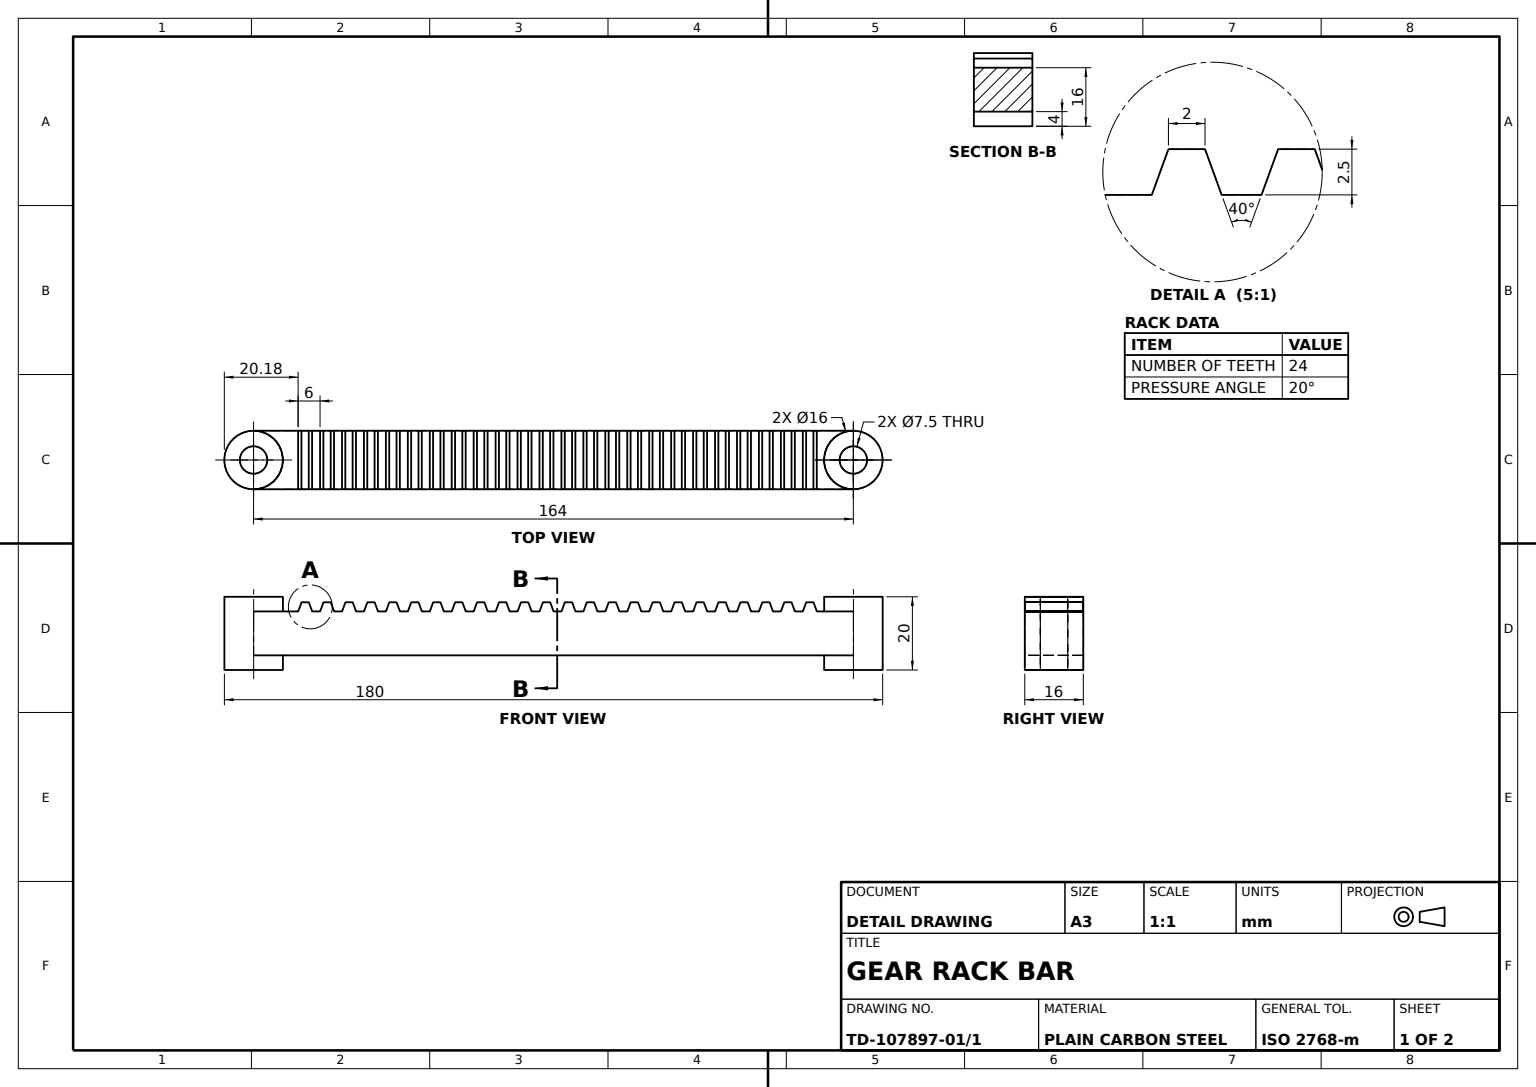
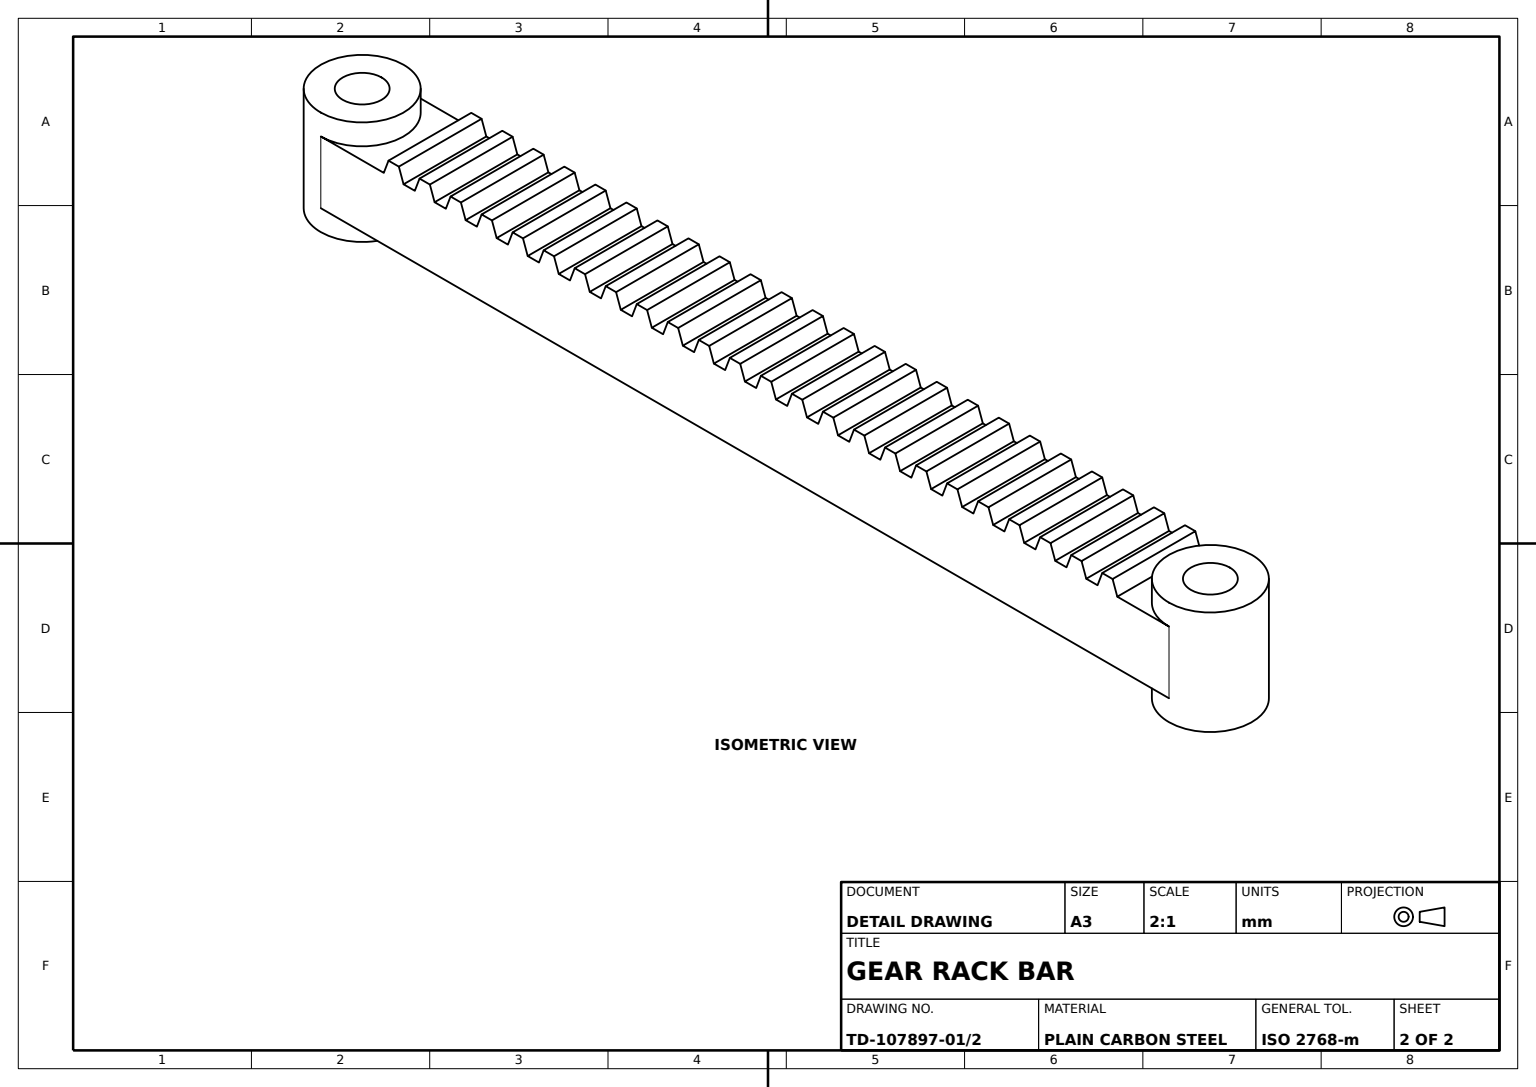
solid
v1 (21.090074,18.5,8)
v2 (21.090074,18.5,-8)
e1 v1 v2 LINE
v3 (20.180149,16,-8)
e2 v2 v3 LINE
v4 (20.180149,16,8)
e3 v4 v3 LINE
e4 v1 v4 LINE
face PLANE(AX(P(12.677219,-4.61413,8),D(0.939692621,-0.342020143,0),D(0.342020143,0.939692621,0))) rev [e1 e2 -e3 -e4]
v5 (-12,16,8)
v6 (-12.909926,18.5,8)
e5 v5 v6 LINE
v7 (-12,16,-8)
e6 v5 v7 LINE
v8 (-12.909926,18.5,-8)
e7 v7 v8 LINE
e8 v6 v8 LINE
face PLANE(AX(P(-5.453966,-1.985081,8),D(-0.939692621,-0.342020143,0),D(0.342020143,-0.939692621,0))) rev [-e5 e6 e7 -e8]
v9 (42,16,8)
v10 (42,16,-8)
e9 v9 v10 LINE
v11 (41.090074,18.5,-8)
e10 v10 v11 LINE
v12 (41.090074,18.5,8)
e11 v12 v11 LINE
e12 v9 v12 LINE
face PLANE(AX(P(42.229234,15.370184,8),D(-0.939692621,-0.342020143,0),D(0.342020143,-0.939692621,0))) rev [e9 e10 -e11 -e12]
v13 (-82,20,8)
v14 (-82,20,-8)
e13 v13 v14 CIRCLE(AX(P(-82,20,0),D(0,1,0),D(0,0,1)),8)
v15 (-82,16,8)
e14 v13 v15 LINE
v16 (-82,16,-8)
e15 v15 v16 CIRCLE(AX(P(-82,16,0),D(0,1,0),D(-1,0,0)),8)
e16 v14 v16 LINE
face CYL(AX(P(-82,20,0),D(0,-1,0),D(0,0,-1)),8) [-e13 e14 e15 -e16]
v17 (18,16,-8)
e17 v17 v3 LINE
v18 (18,16,8)
e18 v18 v17 LINE
e19 v18 v4 LINE
face PLANE(AX(P(0,16,8),D(0,1,0),D(-1,0,0))) [e3 -e17 -e18 e19]
v19 (72,16,8)
v20 (82,16,8)
e20 v19 v20 LINE
v21 (82,16,-8)
e21 v20 v21 CIRCLE(AX(P(82,16,0),D(0,-1,0),D(0,0,1)),8)
v22 (72,16,-8)
e22 v22 v21 LINE
e23 v19 v22 LINE
face PLANE(AX(P(0,16,8),D(0,1,0),D(0,0,1))) [e20 e21 -e22 -e23]
v23 (68.180149,16,8)
v24 (68.180149,16,-8)
e24 v23 v24 LINE
v25 (69.090074,18.5,8)
e25 v25 v23 LINE
v26 (69.090074,18.5,-8)
e26 v25 v26 LINE
e27 v26 v24 LINE
face PLANE(AX(P(55.062286,-20.041033,8),D(0.939692621,-0.342020143,0),D(0.342020143,0.939692621,0))) rev [-e24 -e25 e26 e27]
v27 (82,20,-8)
e28 v27 v21 LINE
v28 (82,20,8)
e29 v28 v27 CIRCLE(AX(P(82,20,0),D(0,1,0),D(0,0,1)),8)
e30 v28 v20 LINE
v29 (82,4,8)
e31 v29 v20 LINE
v30 (82,0,8)
e32 v29 v30 LINE
v31 (82,0,-8)
e33 v30 v31 CIRCLE(AX(P(82,0,0),D(0,1,0),D(0,0,1)),8)
v32 (82,4,-8)
e34 v32 v31 LINE
e35 v32 v21 LINE
face CYL(AX(P(82,20,0),D(0,-1,0),D(0,0,-1)),8) [-e28 -e29 e30 -e31 e32 e33 -e34 e35]
v33 (-8.909926,18.5,8)
v34 (-9.819851,16,8)
e36 v33 v34 LINE
v35 (-8.909926,18.5,-8)
e37 v33 v35 LINE
v36 (-9.819851,16,-8)
e38 v35 v36 LINE
e39 v34 v36 LINE
face PLANE(AX(P(-13.813448,5.027684,8),D(0.939692621,-0.342020143,0),D(0.342020143,0.939692621,0))) rev [-e36 e37 e38 -e39]
e40 v27 v28 CIRCLE(AX(P(82,20,0),D(0,1,0),D(0,0,1)),8)
face CYL(AX(P(82,20,0),D(0,-1,0),D(0,0,-1)),8) [e28 -e21 -e30 -e40]
v37 (-57.819851,16,8)
v38 (-57.819851,16,-8)
e41 v37 v38 LINE
v39 (-56.909926,18.5,8)
e42 v39 v37 LINE
v40 (-56.909926,18.5,-8)
e43 v39 v40 LINE
e44 v40 v38 LINE
face PLANE(AX(P(-56.198514,20.454586,8),D(0.939692621,-0.342020143,0),D(0.342020143,0.939692621,0))) rev [-e41 -e42 e43 e44]
v41 (12,16,-8)
v42 (11.090074,18.5,-8)
e45 v41 v42 LINE
v43 (11.090074,18.5,8)
e46 v43 v42 LINE
v44 (12,16,8)
e47 v44 v43 LINE
e48 v44 v41 LINE
face PLANE(AX(P(15.738568,5.72837,8),D(-0.939692621,-0.342020143,0),D(0.342020143,-0.939692621,0))) rev [e45 -e46 -e47 e48]
v45 (-54,16,-8)
v46 (-54.909926,18.5,-8)
e49 v45 v46 LINE
v47 (-54.909926,18.5,8)
e50 v47 v46 LINE
v48 (-54,16,8)
e51 v48 v47 LINE
e52 v48 v45 LINE
face PLANE(AX(P(-42.540899,-15.483621,8),D(-0.939692621,-0.342020143,0),D(0.342020143,-0.939692621,0))) rev [e49 -e50 -e51 e52]
v49 (30,16,8)
v50 (30,16,-8)
e53 v49 v50 LINE
v51 (29.090074,18.5,-8)
e54 v50 v51 LINE
v52 (29.090074,18.5,8)
e55 v52 v51 LINE
e56 v49 v52 LINE
face PLANE(AX(P(31.632968,11.513459,8),D(-0.939692621,-0.342020143,0),D(0.342020143,-0.939692621,0))) rev [e53 e54 -e55 -e56]
v53 (32.180149,16,8)
v54 (32.180149,16,-8)
e57 v53 v54 LINE
v55 (33.090074,18.5,8)
e58 v55 v53 LINE
v56 (33.090074,18.5,-8)
e59 v55 v56 LINE
e60 v56 v54 LINE
face PLANE(AX(P(23.273486,-8.470856,8),D(0.939692621,-0.342020143,0),D(0.342020143,0.939692621,0))) rev [-e57 -e58 e59 e60]
v57 (9.090074,18.5,8)
v58 (8.180149,16,8)
e61 v57 v58 LINE
v59 (9.090074,18.5,-8)
e62 v57 v59 LINE
v60 (8.180149,16,-8)
e63 v59 v60 LINE
e64 v58 v60 LINE
face PLANE(AX(P(2.080952,-0.757405,8),D(0.939692621,-0.342020143,0),D(0.342020143,0.939692621,0))) rev [-e61 e62 e63 -e64]
e65 v29 v32 CIRCLE(AX(P(82,4,0),D(0,-1,0),D(0,0,1)),8)
v61 (-82,4,8)
e66 v61 v29 LINE
v62 (-82,4,-8)
e67 v61 v62 CIRCLE(AX(P(-82,4,0),D(0,1,0),D(0,0,1)),8)
e68 v62 v32 LINE
face PLANE(AX(P(0,4,8),D(0,1,0),D(0,0,1))) rev [-e65 -e66 e67 e68]
v63 (82,20,-3.75)
v64 (82,20,3.75)
e69 v63 v64 CIRCLE(AX(P(82,20,0),D(0,1,0),D(0,0,1)),3.75)
v65 (82,0,3.75)
e70 v64 v65 LINE
v66 (82,0,-3.75)
e71 v66 v65 CIRCLE(AX(P(82,0,0),D(0,1,0),D(0,0,1)),3.75)
e72 v63 v66 LINE
face CYL(AX(P(82,20,0),D(0,-1,0),D(0,0,-1)),3.75) rev [e69 e70 -e71 -e72]
v67 (60,16,-8)
v68 (62.180149,16,-8)
e73 v67 v68 LINE
v69 (60,16,8)
e74 v69 v67 LINE
v70 (62.180149,16,8)
e75 v69 v70 LINE
e76 v70 v68 LINE
face PLANE(AX(P(0,16,8),D(0,1,0),D(-1,0,0))) [-e73 -e74 e75 e76]
v71 (36,16,8)
v72 (38.180149,16,8)
e77 v71 v72 LINE
v73 (38.180149,16,-8)
e78 v72 v73 LINE
v74 (36,16,-8)
e79 v74 v73 LINE
e80 v71 v74 LINE
face PLANE(AX(P(0,16,8),D(0,1,0),D(-1,0,0))) [e77 e78 -e79 -e80]
v75 (-48.909926,18.5,8)
v76 (-48.909926,18.5,-8)
e81 v75 v76 LINE
v77 (-48,16,8)
e82 v77 v75 LINE
v78 (-48,16,-8)
e83 v77 v78 LINE
e84 v78 v76 LINE
face PLANE(AX(P(-37.242766,-13.555258,8),D(-0.939692621,-0.342020143,0),D(0.342020143,-0.939692621,0))) rev [-e81 -e82 e83 e84]
v79 (-45.819851,16,8)
e85 v77 v79 LINE
v80 (-45.819851,16,-8)
e86 v79 v80 LINE
e87 v78 v80 LINE
face PLANE(AX(P(0,16,8),D(0,1,0),D(-1,0,0))) [-e83 e85 e86 -e87]
v81 (26.180149,16,8)
v82 (26.180149,16,-8)
e88 v81 v82 LINE
v83 (27.090074,18.5,8)
e89 v83 v81 LINE
v84 (27.090074,18.5,-8)
e90 v83 v84 LINE
e91 v84 v82 LINE
face PLANE(AX(P(17.975352,-6.542493,8),D(0.939692621,-0.342020143,0),D(0.342020143,0.939692621,0))) rev [-e88 -e89 e90 e91]
v85 (-14.909926,18.5,-8)
v86 (-15.819851,16,-8)
e92 v85 v86 LINE
v87 (-15.819851,16,8)
e93 v87 v86 LINE
v88 (-14.909926,18.5,8)
e94 v88 v87 LINE
e95 v88 v85 LINE
face PLANE(AX(P(-19.111581,6.956047,8),D(0.939692621,-0.342020143,0),D(0.342020143,0.939692621,0))) rev [e92 -e93 -e94 e95]
v89 (17.090074,18.5,-8)
e96 v17 v89 LINE
v90 (17.090074,18.5,8)
e97 v90 v89 LINE
e98 v18 v90 LINE
face PLANE(AX(P(21.036701,7.656733,8),D(-0.939692621,-0.342020143,0),D(0.342020143,-0.939692621,0))) rev [e18 e96 -e97 -e98]
e99 v31 v30 CIRCLE(AX(P(82,0,0),D(0,1,0),D(0,0,1)),8)
e100 v65 v66 CIRCLE(AX(P(82,0,0),D(0,1,0),D(0,0,1)),3.75)
face PLANE(AX(P(82,0,0),D(0,1,0),D(0,0,1))) rev [-e33 -e99] [e100 e71]
v91 (-27.819851,16,8)
v92 (-27.819851,16,-8)
e101 v91 v92 LINE
v93 (-26.909926,18.5,8)
e102 v93 v91 LINE
v94 (-26.909926,18.5,-8)
e103 v93 v94 LINE
e104 v94 v92 LINE
face PLANE(AX(P(-29.707848,10.812772,8),D(0.939692621,-0.342020143,0),D(0.342020143,0.939692621,0))) rev [-e101 -e102 e103 e104]
v95 (53.090074,18.5,8)
v96 (53.090074,18.5,-8)
e105 v95 v96 LINE
v97 (51.090074,18.5,-8)
e106 v96 v97 LINE
v98 (51.090074,18.5,8)
e107 v98 v97 LINE
e108 v95 v98 LINE
face PLANE(AX(P(0,18.5,8),D(0,-1,0),D(0,0,-1))) rev [e105 e106 -e107 -e108]
v99 (-50.909926,18.5,8)
v100 (-51.819851,16,8)
e109 v99 v100 LINE
v101 (-50.909926,18.5,-8)
e110 v99 v101 LINE
v102 (-51.819851,16,-8)
e111 v101 v102 LINE
e112 v100 v102 LINE
face PLANE(AX(P(-50.900381,18.526224,8),D(0.939692621,-0.342020143,0),D(0.342020143,0.939692621,0))) rev [-e109 e110 e111 -e112]
v103 (-44.909926,18.5,8)
v104 (-44.909926,18.5,-8)
e113 v103 v104 LINE
e114 v104 v80 LINE
e115 v103 v79 LINE
face PLANE(AX(P(-45.602248,16.597861,8),D(0.939692621,-0.342020143,0),D(0.342020143,0.939692621,0))) rev [e113 e114 -e86 -e115]
v105 (39.090074,18.5,-8)
e116 v11 v105 LINE
v106 (39.090074,18.5,8)
e117 v106 v105 LINE
e118 v12 v106 LINE
face PLANE(AX(P(0,18.5,8),D(0,-1,0),D(0,0,-1))) rev [e11 e116 -e117 -e118]
v107 (-18,16,8)
e119 v107 v87 LINE
v108 (-18,16,-8)
e120 v108 v86 LINE
e121 v107 v108 LINE
face PLANE(AX(P(0,16,8),D(0,1,0),D(-1,0,0))) [e119 e93 -e120 -e121]
v109 (-63.819851,16,8)
v110 (-63.819851,16,-8)
e122 v109 v110 LINE
v111 (-62.909926,18.5,8)
e123 v111 v109 LINE
v112 (-62.909926,18.5,-8)
e124 v111 v112 LINE
e125 v112 v110 LINE
face PLANE(AX(P(-61.496648,22.382949,8),D(0.939692621,-0.342020143,0),D(0.342020143,0.939692621,0))) rev [-e122 -e123 e124 e125]
v113 (44.180149,16,8)
v114 (44.180149,16,-8)
e126 v113 v114 LINE
v115 (45.090074,18.5,8)
e127 v115 v113 LINE
v116 (45.090074,18.5,-8)
e128 v115 v116 LINE
e129 v116 v114 LINE
face PLANE(AX(P(33.869752,-12.327582,8),D(0.939692621,-0.342020143,0),D(0.342020143,0.939692621,0))) rev [-e126 -e127 e128 e129]
v117 (-60.909926,18.5,8)
e130 v117 v111 LINE
v118 (-60.909926,18.5,-8)
e131 v117 v118 LINE
e132 v118 v112 LINE
face PLANE(AX(P(0,18.5,8),D(0,-1,0),D(0,0,-1))) rev [-e124 -e130 e131 e132]
e133 v47 v39 LINE
e134 v46 v40 LINE
face PLANE(AX(P(0,18.5,8),D(0,-1,0),D(0,0,-1))) rev [-e133 e50 e134 -e43]
v119 (35.090074,18.5,8)
e135 v119 v55 LINE
v120 (35.090074,18.5,-8)
e136 v119 v120 LINE
e137 v120 v56 LINE
face PLANE(AX(P(0,18.5,8),D(0,-1,0),D(0,0,-1))) rev [-e59 -e135 e136 e137]
face CYL(AX(P(82,20,0),D(0,-1,0),D(0,0,-1)),8) [-e32 e65 e34 e99]
v121 (-30.909926,18.5,8)
v122 (-30.909926,18.5,-8)
e138 v121 v122 LINE
v123 (-30,16,8)
e139 v123 v121 LINE
v124 (-30,16,-8)
e140 v123 v124 LINE
e141 v124 v122 LINE
face PLANE(AX(P(-21.348366,-7.77017,8),D(-0.939692621,-0.342020143,0),D(0.342020143,-0.939692621,0))) rev [-e138 -e139 e140 e141]
v125 (-38.909926,18.5,-8)
v126 (-39.819851,16,-8)
e142 v125 v126 LINE
v127 (-39.819851,16,8)
e143 v127 v126 LINE
v128 (-38.909926,18.5,8)
e144 v128 v127 LINE
e145 v128 v125 LINE
face PLANE(AX(P(-40.304114,14.669498,8),D(0.939692621,-0.342020143,0),D(0.342020143,0.939692621,0))) rev [e142 -e143 -e144 e145]
v129 (47.090074,18.5,8)
v130 (47.090074,18.5,-8)
e146 v129 v130 LINE
e147 v130 v116 LINE
e148 v129 v115 LINE
face PLANE(AX(P(0,18.5,8),D(0,-1,0),D(0,0,-1))) rev [e146 e147 -e128 -e148]
e149 v64 v63 CIRCLE(AX(P(82,20,0),D(0,1,0),D(0,0,1)),3.75)
face CYL(AX(P(82,20,0),D(0,-1,0),D(0,0,-1)),3.75) rev [-e70 e149 e72 -e100]
v131 (-42.909926,18.5,8)
e150 v131 v103 LINE
v132 (-42.909926,18.5,-8)
e151 v131 v132 LINE
e152 v132 v104 LINE
face PLANE(AX(P(0,18.5,8),D(0,-1,0),D(0,0,-1))) rev [-e150 e151 e152 -e113]
v133 (14.180149,16,8)
v134 (14.180149,16,-8)
e153 v133 v134 LINE
v135 (15.090074,18.5,8)
e154 v135 v133 LINE
v136 (15.090074,18.5,-8)
e155 v135 v136 LINE
e156 v136 v134 LINE
face PLANE(AX(P(7.379086,-2.685768,8),D(0.939692621,-0.342020143,0),D(0.342020143,0.939692621,0))) rev [-e153 -e154 e155 e156]
v137 (50.180149,16,-8)
e157 v97 v137 LINE
v138 (50.180149,16,8)
e158 v138 v137 LINE
e159 v98 v138 LINE
face PLANE(AX(P(39.167886,-14.255945,8),D(0.939692621,-0.342020143,0),D(0.342020143,0.939692621,0))) rev [e107 e157 -e158 -e159]
v139 (-69.819851,16,-8)
e160 v16 v139 LINE
v140 (-69.819851,16,8)
e161 v15 v140 LINE
e162 v140 v139 LINE
face PLANE(AX(P(0,16,8),D(0,1,0),D(-1,0,0))) [-e160 -e15 e161 e162]
v141 (-82,0,-8)
e163 v62 v141 LINE
v142 (-82,0,8)
e164 v141 v142 CIRCLE(AX(P(-82,0,0),D(0,1,0),D(0,0,1)),8)
e165 v61 v142 LINE
e166 v61 v15 LINE
e167 v14 v13 CIRCLE(AX(P(-82,20,0),D(0,1,0),D(0,0,1)),8)
e168 v62 v16 LINE
face CYL(AX(P(-82,20,0),D(0,-1,0),D(0,0,-1)),8) [e163 e164 -e165 e166 -e14 -e167 e16 -e168]
e169 v106 v72 LINE
e170 v105 v73 LINE
face PLANE(AX(P(28.571619,-10.399219,8),D(0.939692621,-0.342020143,0),D(0.342020143,0.939692621,0))) rev [-e78 -e169 e117 e170]
v143 (-66.909926,18.5,8)
v144 (-66.909926,18.5,-8)
e171 v143 v144 LINE
v145 (-68.909926,18.5,-8)
e172 v144 v145 LINE
v146 (-68.909926,18.5,8)
e173 v146 v145 LINE
e174 v143 v146 LINE
face PLANE(AX(P(0,18.5,8),D(0,-1,0),D(0,0,-1))) rev [e171 e172 -e173 -e174]
v147 (-42,16,8)
e175 v147 v127 LINE
e176 v147 v131 LINE
e177 v75 v99 LINE
e178 v48 v100 LINE
v148 (-60,16,8)
e179 v148 v37 LINE
e180 v148 v117 LINE
v149 (-66,16,8)
e181 v149 v109 LINE
e182 v149 v143 LINE
e183 v146 v140 LINE
v150 (71.090074,18.5,8)
e184 v19 v150 LINE
e185 v150 v25 LINE
v151 (66,16,8)
e186 v151 v23 LINE
v152 (65.090074,18.5,8)
e187 v151 v152 LINE
v153 (63.090074,18.5,8)
e188 v152 v153 LINE
e189 v153 v70 LINE
v154 (59.090074,18.5,8)
e190 v69 v154 LINE
v155 (57.090074,18.5,8)
e191 v154 v155 LINE
v156 (56.180149,16,8)
e192 v155 v156 LINE
v157 (54,16,8)
e193 v157 v156 LINE
e194 v157 v95 LINE
v158 (48,16,8)
e195 v158 v138 LINE
e196 v158 v129 LINE
e197 v9 v113 LINE
e198 v71 v119 LINE
e199 v49 v53 LINE
e200 v52 v83 LINE
v159 (24,16,8)
e201 v159 v81 LINE
v160 (23.090074,18.5,8)
e202 v159 v160 LINE
e203 v160 v1 LINE
e204 v90 v135 LINE
e205 v44 v133 LINE
e206 v43 v57 LINE
v161 (6,16,8)
e207 v161 v58 LINE
v162 (5.090074,18.5,8)
e208 v161 v162 LINE
v163 (3.090074,18.5,8)
e209 v162 v163 LINE
v164 (2.180149,16,8)
e210 v163 v164 LINE
v165 (0,16,8)
e211 v165 v164 LINE
v166 (-0.909926,18.5,8)
e212 v165 v166 LINE
v167 (-2.909926,18.5,8)
e213 v166 v167 LINE
v168 (-3.819851,16,8)
e214 v167 v168 LINE
v169 (-6,16,8)
e215 v169 v168 LINE
v170 (-6.909926,18.5,8)
e216 v169 v170 LINE
e217 v170 v33 LINE
e218 v5 v34 LINE
e219 v6 v88 LINE
v171 (-18.909926,18.5,8)
e220 v107 v171 LINE
v172 (-20.909926,18.5,8)
e221 v171 v172 LINE
v173 (-21.819851,16,8)
e222 v172 v173 LINE
v174 (-24,16,8)
e223 v174 v173 LINE
v175 (-24.909926,18.5,8)
e224 v174 v175 LINE
e225 v175 v93 LINE
e226 v123 v91 LINE
v176 (-32.909926,18.5,8)
e227 v121 v176 LINE
v177 (-33.819851,16,8)
e228 v176 v177 LINE
v178 (-36,16,8)
e229 v178 v177 LINE
v179 (-36.909926,18.5,8)
e230 v178 v179 LINE
e231 v179 v128 LINE
face PLANE(AX(P(0,0,8),D(0,0,1),D(1,0,0))) [-e175 e176 e150 e115 -e85 e82 e177 e109 -e178 e51 e133 e42 -e179 e180 e130 e123 -e181 e182 e174 e183 -e161 -e166 e66 e31 -e20 e184 e185 e25 -e186 e187 e188 e189 -e75 e190 e191 e192 -e193 e194 e108 e159 -e195 e196 e148 e127 -e197 e12 e118 e169 -e77 e198 e135 e58 -e199 e56 e200 e89 -e201 e202 e203 e4 -e19 e98 e204 e154 -e205 e47 e206 e61 -e207 e208 e209 e210 -e211 e212 e213 e214 -e215 e216 e217 e36 -e218 e5 e219 e94 -e119 e220 e221 e222 -e223 e224 e225 e102 -e226 e139 e227 e228 -e229 e230 e231 e144]
v180 (65.090074,18.5,-8)
e232 v152 v180 LINE
v181 (63.090074,18.5,-8)
e233 v180 v181 LINE
e234 v153 v181 LINE
face PLANE(AX(P(0,18.5,8),D(0,-1,0),D(1,0,0))) rev [e232 e233 -e234 -e188]
e235 v8 v85 LINE
face PLANE(AX(P(0,18.5,8),D(0,-1,0),D(0,0,-1))) rev [-e95 -e219 e8 e235]
v182 (6,16,-8)
e236 v182 v60 LINE
e237 v161 v182 LINE
face PLANE(AX(P(0,16,8),D(0,1,0),D(-1,0,0))) [e207 e64 -e236 -e237]
v183 (66,16,-8)
e238 v183 v24 LINE
e239 v151 v183 LINE
face PLANE(AX(P(0,16,8),D(0,1,0),D(0,0,1))) [e24 -e238 -e239 e186]
e240 v45 v102 LINE
face PLANE(AX(P(0,16,8),D(0,1,0),D(-1,0,0))) [e178 e112 -e240 -e52]
e241 v50 v54 LINE
face PLANE(AX(P(0,16,8),D(0,1,0),D(-1,0,0))) [-e241 -e53 e199 e57]
v184 (-82,20,-3.75)
v185 (-82,20,3.75)
e242 v184 v185 CIRCLE(AX(P(-82,20,0),D(0,1,0),D(0,0,1)),3.75)
e243 v185 v184 CIRCLE(AX(P(-82,20,0),D(0,1,0),D(0,0,1)),3.75)
face PLANE(AX(P(-82,20,0),D(0,1,0),D(0,0,1))) [-e242 -e243] [e167 e13]
v186 (48,16,-8)
e244 v158 v186 LINE
e245 v186 v130 LINE
face PLANE(AX(P(47.527368,17.298547,8),D(-0.939692621,-0.342020143,0),D(0.342020143,-0.939692621,0))) rev [e244 e245 -e146 -e196]
v187 (0,16,-8)
e246 v165 v187 LINE
v188 (-0.909926,18.5,-8)
e247 v187 v188 LINE
e248 v166 v188 LINE
face PLANE(AX(P(5.142301,1.871644,8),D(-0.939692621,-0.342020143,0),D(0.342020143,-0.939692621,0))) rev [-e212 e246 e247 -e248]
v189 (5.090074,18.5,-8)
e249 v162 v189 LINE
v190 (3.090074,18.5,-8)
e250 v189 v190 LINE
e251 v163 v190 LINE
face PLANE(AX(P(0,18.5,8),D(0,-1,0),D(0,0,-1))) rev [e249 e250 -e251 -e209]
v191 (24,16,-8)
e252 v191 v82 LINE
e253 v159 v191 LINE
face PLANE(AX(P(0,16,8),D(0,1,0),D(-1,0,0))) [e88 -e252 -e253 e201]
v192 (-36.909926,18.5,-8)
e254 v179 v192 LINE
e255 v192 v125 LINE
face PLANE(AX(P(0,18.5,8),D(0,-1,0),D(0,0,-1))) rev [e254 e255 -e145 -e231]
e256 v142 v141 CIRCLE(AX(P(-82,0,0),D(0,1,0),D(0,0,1)),8)
face CYL(AX(P(-82,20,0),D(0,-1,0),D(0,0,-1)),8) [-e67 e165 e256 -e163]
v193 (-42,16,-8)
e257 v193 v132 LINE
e258 v147 v193 LINE
face PLANE(AX(P(-31.944632,-11.626895,8),D(-0.939692621,-0.342020143,0),D(0.342020143,-0.939692621,0))) rev [e257 -e151 -e176 e258]
v194 (2.180149,16,-8)
e259 v190 v194 LINE
e260 v164 v194 LINE
face PLANE(AX(P(-3.217181,1.170958,8),D(0.939692621,-0.342020143,0),D(0.342020143,0.939692621,0))) rev [-e210 e251 e259 -e260]
v195 (56.180149,16,-8)
e261 v156 v195 LINE
v196 (54,16,-8)
e262 v196 v195 LINE
e263 v157 v196 LINE
face PLANE(AX(P(0,16,8),D(0,1,0),D(-1,0,0))) [e261 -e262 -e263 e193]
e264 v182 v189 LINE
face PLANE(AX(P(10.440434,3.800007,8),D(-0.939692621,-0.342020143,0),D(0.342020143,-0.939692621,0))) rev [e264 -e249 -e208 e237]
v197 (-82,0,-3.75)
e265 v184 v197 LINE
v198 (-82,0,3.75)
e266 v198 v197 CIRCLE(AX(P(-82,0,0),D(0,1,0),D(0,0,1)),3.75)
e267 v185 v198 LINE
face CYL(AX(P(-82,20,0),D(0,-1,0),D(0,0,-1)),3.75) rev [e265 -e266 -e267 e243]
e268 v187 v194 LINE
face PLANE(AX(P(0,16,8),D(0,1,0),D(-1,0,0))) [e211 e260 -e268 -e246]
v199 (23.090074,18.5,-8)
e269 v199 v2 LINE
e270 v160 v199 LINE
face PLANE(AX(P(0,18.5,8),D(0,-1,0),D(0,0,-1))) rev [e269 -e1 -e203 e270]
v200 (-18.909926,18.5,-8)
v201 (-20.909926,18.5,-8)
e271 v200 v201 LINE
e272 v172 v201 LINE
e273 v171 v200 LINE
face PLANE(AX(P(0,18.5,8),D(0,-1,0),D(0,0,-1))) rev [e271 -e272 -e221 e273]
v202 (-2.909926,18.5,-8)
e274 v188 v202 LINE
e275 v167 v202 LINE
face PLANE(AX(P(0,18.5,8),D(0,-1,0),D(0,0,-1))) rev [-e213 e248 e274 -e275]
v203 (-33.819851,16,-8)
e276 v177 v203 LINE
v204 (-36,16,-8)
e277 v204 v203 LINE
e278 v178 v204 LINE
face PLANE(AX(P(0,16,8),D(0,1,0),D(-1,0,0))) [e229 e276 -e277 -e278]
e279 v124 v92 LINE
face PLANE(AX(P(0,16,8),D(0,1,0),D(-1,0,0))) [e226 e101 -e279 -e140]
v205 (-60,16,-8)
e280 v205 v38 LINE
e281 v148 v205 LINE
face PLANE(AX(P(0,16,8),D(0,1,0),D(-1,0,0))) [e179 e41 -e280 -e281]
e282 v42 v59 LINE
face PLANE(AX(P(0,18.5,8),D(0,-1,0),D(0,0,-1))) rev [e46 e282 -e62 -e206]
e283 v7 v36 LINE
face PLANE(AX(P(0,16,8),D(0,1,0),D(-1,0,0))) [e218 e39 -e283 -e6]
e284 v191 v199 LINE
face PLANE(AX(P(26.334834,9.585096,8),D(-0.939692621,-0.342020143,0),D(0.342020143,-0.939692621,0))) rev [-e270 -e202 e253 e284]
e285 v183 v180 LINE
face PLANE(AX(P(63.421768,23.083636,8),D(-0.939692621,-0.342020143,0),D(0.342020143,-0.939692621,0))) rev [e239 e285 -e232 -e187]
v206 (-24.909926,18.5,-8)
e286 v175 v206 LINE
e287 v206 v94 LINE
face PLANE(AX(P(0,18.5,8),D(0,-1,0),D(0,0,-1))) rev [-e103 -e225 e286 e287]
e288 v108 v200 LINE
face PLANE(AX(P(-10.752099,-3.913444,8),D(-0.939692621,-0.342020143,0),D(0.342020143,-0.939692621,0))) rev [e121 e288 -e273 -e220]
v207 (57.090074,18.5,-8)
e289 v155 v207 LINE
e290 v207 v195 LINE
face PLANE(AX(P(44.466019,-16.184307,8),D(0.939692621,-0.342020143,0),D(0.342020143,0.939692621,0))) rev [e289 e290 -e261 -e192]
e291 v181 v68 LINE
face PLANE(AX(P(49.764152,-18.11267,8),D(0.939692621,-0.342020143,0),D(0.342020143,0.939692621,0))) rev [e234 e291 -e76 -e189]
e292 v145 v139 LINE
face PLANE(AX(P(-66.794781,24.311312,8),D(0.939692621,-0.342020143,0),D(0.342020143,0.939692621,0))) rev [-e183 e173 e292 -e162]
v208 (-21.819851,16,-8)
e293 v201 v208 LINE
e294 v173 v208 LINE
face PLANE(AX(P(-24.409714,8.884409,8),D(0.939692621,-0.342020143,0),D(0.342020143,0.939692621,0))) rev [e293 -e294 -e222 e272]
e295 v196 v96 LINE
face PLANE(AX(P(52.825501,19.22691,8),D(-0.939692621,-0.342020143,0),D(0.342020143,-0.939692621,0))) rev [e295 -e105 -e194 e263]
e296 v193 v126 LINE
face PLANE(AX(P(0,16,8),D(0,1,0),D(-1,0,0))) [-e258 e175 e143 -e296]
v209 (-66,16,-8)
e297 v149 v209 LINE
e298 v209 v110 LINE
face PLANE(AX(P(0,16,8),D(0,1,0),D(-1,0,0))) [-e297 e181 e122 -e298]
v210 (71.090074,18.5,-8)
e299 v150 v210 LINE
e300 v22 v210 LINE
face PLANE(AX(P(68.719901,25.011998,8),D(-0.939692621,-0.342020143,0),D(0.342020143,-0.939692621,0))) rev [-e299 -e184 e23 e300]
e301 v204 v192 LINE
face PLANE(AX(P(-26.646499,-9.698533,8),D(-0.939692621,-0.342020143,0),D(0.342020143,-0.939692621,0))) rev [-e230 e278 e301 -e254]
e302 v51 v84 LINE
face PLANE(AX(P(0,18.5,8),D(0,-1,0),D(0,0,-1))) rev [-e90 -e200 e55 e302]
e303 v74 v120 LINE
face PLANE(AX(P(36.931101,13.441821,8),D(-0.939692621,-0.342020143,0),D(0.342020143,-0.939692621,0))) rev [e80 e303 -e136 -e198]
face PLANE(AX(P(82,20,0),D(0,1,0),D(0,0,1))) [-e149 -e69] [e29 e40]
v211 (-32.909926,18.5,-8)
e304 v176 v211 LINE
e305 v211 v203 LINE
face PLANE(AX(P(-35.005981,12.741135,8),D(0.939692621,-0.342020143,0),D(0.342020143,0.939692621,0))) rev [e304 e305 -e276 -e228]
e306 v89 v136 LINE
face PLANE(AX(P(0,18.5,8),D(0,-1,0),D(0,0,-1))) rev [e306 -e155 -e204 e97]
e307 v10 v114 LINE
face PLANE(AX(P(0,16,8),D(0,1,0),D(-1,0,0))) [-e9 e197 e126 -e307]
v212 (-6,16,-8)
v213 (-6.909926,18.5,-8)
e308 v212 v213 LINE
e309 v170 v213 LINE
e310 v169 v212 LINE
face PLANE(AX(P(-0.155832,-0.056718,8),D(-0.939692621,-0.342020143,0),D(0.342020143,-0.939692621,0))) rev [e308 -e309 -e216 e310]
e311 v210 v26 LINE
face PLANE(AX(P(0,18.5,8),D(0,-1,0),D(0,0,-1))) rev [e311 -e26 -e185 e299]
v214 (59.090074,18.5,-8)
e312 v214 v207 LINE
e313 v154 v214 LINE
face PLANE(AX(P(0,18.5,8),D(0,-1,0),D(0,0,-1))) rev [e312 -e289 -e191 e313]
e314 v209 v144 LINE
e315 v205 v118 LINE
e316 v76 v101 LINE
e317 v122 v211 LINE
v215 (-24,16,-8)
e318 v215 v206 LINE
e319 v215 v208 LINE
e320 v213 v35 LINE
v216 (-3.819851,16,-8)
e321 v212 v216 LINE
e322 v202 v216 LINE
e323 v41 v134 LINE
e324 v186 v137 LINE
e325 v67 v214 LINE
face PLANE(AX(P(0,0,-8),D(0,0,1),D(1,0,0))) rev [e238 -e27 -e311 -e300 e22 -e35 -e68 e168 e160 -e292 -e172 -e314 e298 -e125 -e132 -e315 e280 -e44 -e134 -e49 e240 -e111 -e316 -e84 e87 -e114 -e152 -e257 e296 -e142 -e255 -e301 e277 -e305 -e317 -e141 e279 -e104 -e287 -e318 e319 -e293 -e271 -e288 e120 -e92 -e235 -e7 e283 -e38 -e320 -e308 e321 -e322 -e274 -e247 e268 -e259 -e250 -e264 e236 -e63 -e282 -e45 e323 -e156 -e306 -e96 e17 -e2 -e269 -e284 e252 -e91 -e302 -e54 e241 -e60 -e137 -e303 e79 -e170 -e116 -e10 e307 -e129 -e147 -e245 e324 -e157 -e106 -e295 e262 -e290 -e312 -e325 e73 -e291 -e233 -e285]
face PLANE(AX(P(0,16,8),D(0,1,0),D(-1,0,0))) [e158 -e324 -e244 e195]
face PLANE(AX(P(0,18.5,8),D(0,-1,0),D(0,0,-1))) rev [e316 -e110 -e177 e81]
e326 v197 v198 CIRCLE(AX(P(-82,0,0),D(0,1,0),D(0,0,1)),3.75)
face PLANE(AX(P(-82,0,0),D(0,1,0),D(0,0,1))) rev [-e164 -e256] [e326 e266]
face PLANE(AX(P(-47.839032,-17.411984,8),D(-0.939692621,-0.342020143,0),D(0.342020143,-0.939692621,0))) rev [e281 e315 -e131 -e180]
face PLANE(AX(P(0,16,8),D(0,1,0),D(-1,0,0))) [e153 -e323 -e48 e205]
face CYL(AX(P(-82,20,0),D(0,-1,0),D(0,0,-1)),3.75) rev [-e326 -e265 e242 e267]
e327 v168 v216 LINE
face PLANE(AX(P(-8.515314,3.099321,8),D(0.939692621,-0.342020143,0),D(0.342020143,0.939692621,0))) rev [-e214 e275 e322 -e327]
e328 v174 v215 LINE
face PLANE(AX(P(-16.050232,-5.841807,8),D(-0.939692621,-0.342020143,0),D(0.342020143,-0.939692621,0))) rev [-e286 -e224 e328 e318]
face PLANE(AX(P(0,18.5,8),D(0,-1,0),D(0,0,-1))) rev [e309 e320 -e37 -e217]
face PLANE(AX(P(0,18.5,8),D(0,-1,0),D(0,0,-1))) rev [e317 -e304 -e227 e138]
face PLANE(AX(P(58.123634,21.155273,8),D(-0.939692621,-0.342020143,0),D(0.342020143,-0.939692621,0))) rev [e74 e325 -e313 -e190]
face PLANE(AX(P(0,16,8),D(0,1,0),D(-1,0,0))) [e294 -e319 -e328 e223]
face PLANE(AX(P(0,16,8),D(0,1,0),D(-1,0,0))) [e327 -e321 -e310 e215]
face PLANE(AX(P(-53.137166,-19.340347,8),D(-0.939692621,-0.342020143,0),D(0.342020143,-0.939692621,0))) rev [e314 -e171 -e182 e297]
